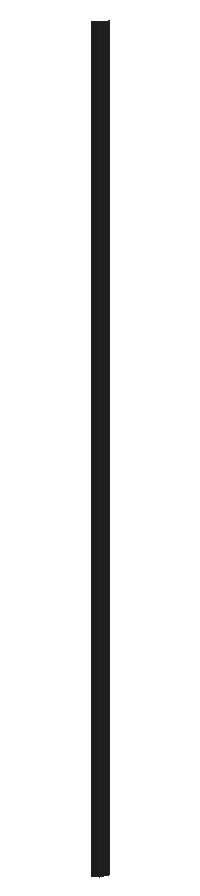
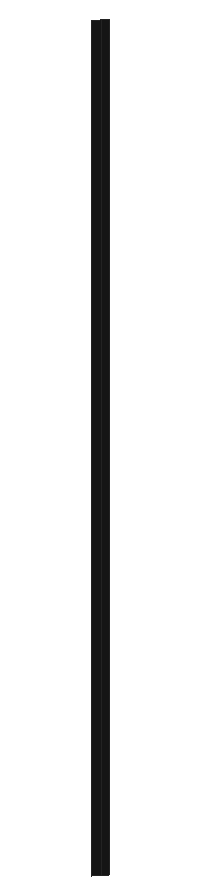
# SketchUp Ruby script. Lengths in inches.
U = 1.inch
M = Sketchup.active_model
def pt(a) = Geom::Point3d.new(a.map { |v| v * U })
def face(e, loops, mat)
  f = e.add_face(loops[0].map { |a| pt(a) })
  loops[1..].each { |l| e.add_face(l.map { |a| pt(a) }).erase! }
  f.material = f.back_material = mat if mat
  f
end
# faces: each face lists its corners as indices into pts; further lists are holes
def faces(e, pts, list, mat = nil) = list.each { |f| face(e, (f[0].is_a?(Array) ? f : [f]).map { |l| l.map { |i| pts[i] } }, mat) }
# xy, xz, yz: faces in a plane at the given z, y or x. An outline is a flat list of corners, or four numbers for a rectangle; further outlines are holes
def ring(l) = l.size == 4 ? [[l[0], l[1]], [l[2], l[1]], [l[2], l[3]], [l[0], l[3]]] : l.each_slice(2).to_a
def flat(e, list, mat, &to3) = list.each { |f| face(e, (f[0].is_a?(Array) ? f : [f]).map { |l| ring(l).map { |u, v| to3.(u, v) } }, mat) }
def xy(e, z, list, mat = nil) = flat(e, list, mat) { |x, y| [x, y, z] }
def xz(e, y, list, mat = nil) = flat(e, list, mat) { |x, z| [x, y, z] }
def yz(e, x, list, mat = nil) = flat(e, list, mat) { |y, z| [x, y, z] }
def lines(e, pts, list) = list.each { |a, b| e.add_line(pt(pts[a]), pt(pts[b])) }
# prism: a flat outline (further loops are holes) pulled along v
def prism(e, loops, v, mat = nil)
  f = face(e, loops, mat); d = Geom::Vector3d.new(v.map { |x| x * U })
  f.pushpull(f.normal.samedirection?(d) ? d.length : -d.length)
end
def box(e, o, s, mat = nil) = prism(e, [[o, [o[0] + s[0], o[1], o[2]], [o[0] + s[0], o[1] + s[1], o[2]], [o[0], o[1] + s[1], o[2]]]], [0, 0, s[2]], mat)
def at(x, y, z, deg = 0) = Geom::Transformation.translation(pt([x, y, z])) * Geom::Transformation.rotation(ORIGIN, Z_AXIS, deg.degrees)
def axes(o, x, y, z) = Geom::Transformation.new([*x, 0, *y, 0, *z, 0, *pt(o).to_a, 1])
def part(name) = M.definitions.add(name)
# library, detail: a bought-in or finely detailed component or shape, given as its bounding box
def library(name, o, s) = part(name).tap { |d| box(d.entities, o, s) }
def detail(e, o, s) = box(e.add_group.entities, o, s)
def put(e, d, t, mat = nil) = e.add_instance(d, t).tap { |i| i.material = mat if mat }
def group(e, t, mat = nil) = e.add_group.tap { |g| g.transformation = t; g.material = mat if mat }.entities
root = M.entities
M.materials.add("[0136_Charcoal]").color = [35, 35, 35]
p = [[263.99,227.61,142.6875],[264.18,227.76,142.6875],[264.18,227.76,171.3125],[263.99,227.61,171.3125],[264.33,227.96,142.6875],[264.33,227.96,171.3125]]
faces(root,p,[[0,1,2,3],[1,4,5,2]],"[0136_Charcoal]")
